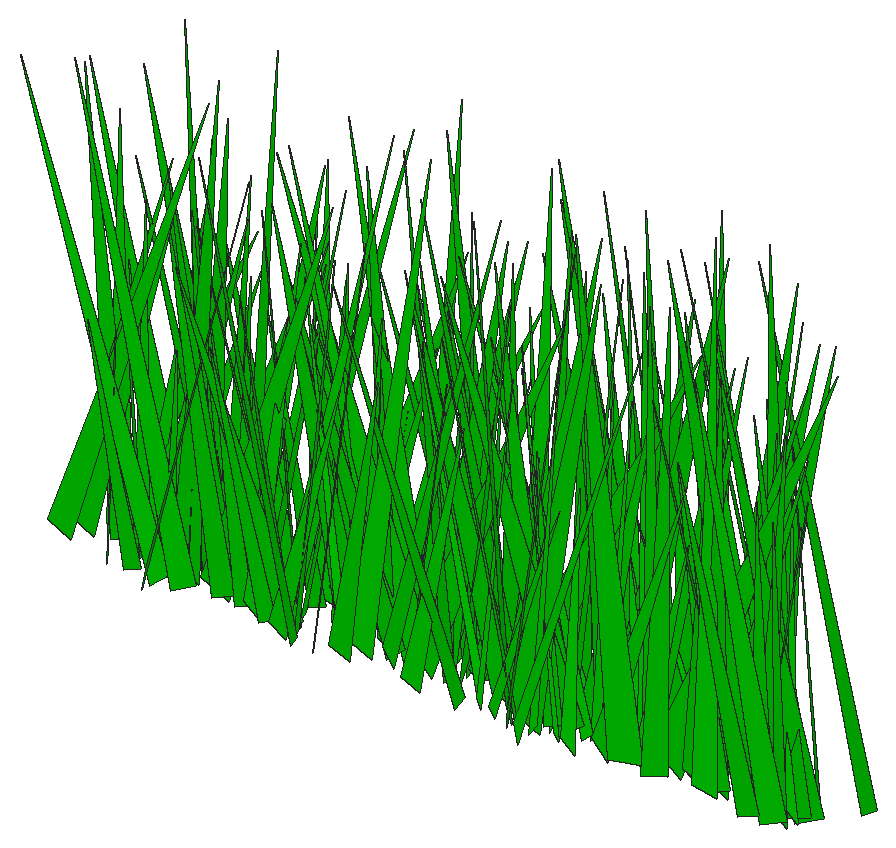
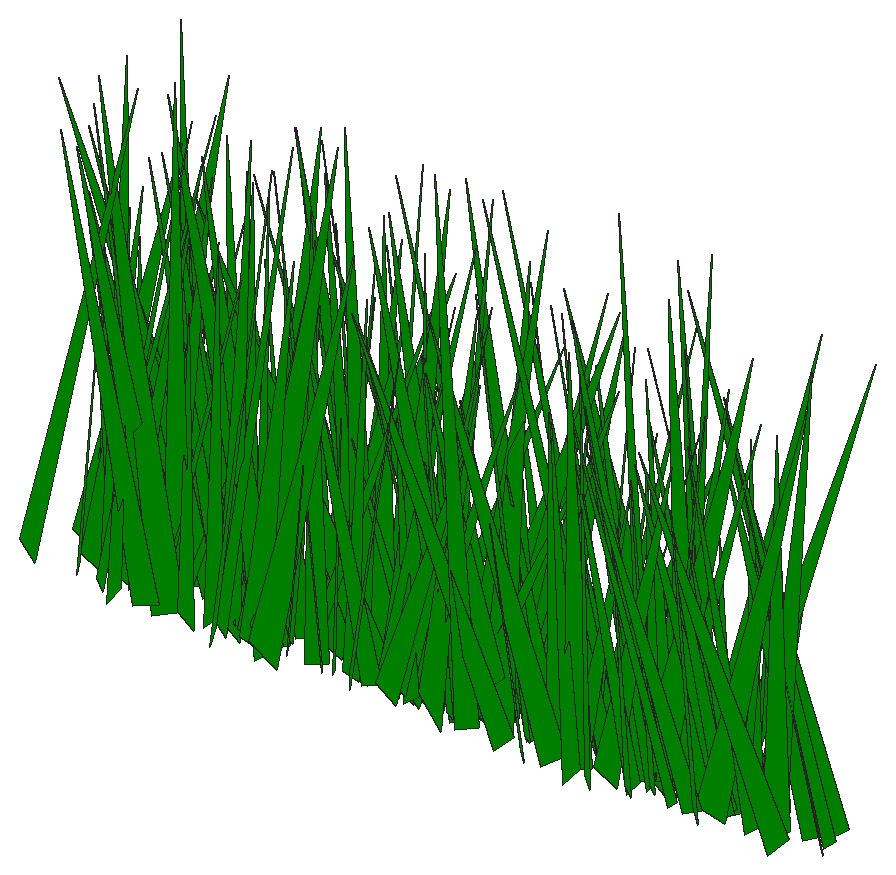
# SketchUp Ruby script. Lengths in inches.
U = 1.inch
M = Sketchup.active_model
def pt(a) = Geom::Point3d.new(a.map { |v| v * U })
def face(e, loops, mat)
  f = e.add_face(loops[0].map { |a| pt(a) })
  loops[1..].each { |l| e.add_face(l.map { |a| pt(a) }).erase! }
  f.material = f.back_material = mat if mat
  f
end
# faces: each face lists its corners as indices into pts; further lists are holes
def faces(e, pts, list, mat = nil) = list.each { |f| face(e, (f[0].is_a?(Array) ? f : [f]).map { |l| l.map { |i| pts[i] } }, mat) }
# xy, xz, yz: faces in a plane at the given z, y or x. An outline is a flat list of corners, or four numbers for a rectangle; further outlines are holes
def ring(l) = l.size == 4 ? [[l[0], l[1]], [l[2], l[1]], [l[2], l[3]], [l[0], l[3]]] : l.each_slice(2).to_a
def flat(e, list, mat, &to3) = list.each { |f| face(e, (f[0].is_a?(Array) ? f : [f]).map { |l| ring(l).map { |u, v| to3.(u, v) } }, mat) }
def xy(e, z, list, mat = nil) = flat(e, list, mat) { |x, y| [x, y, z] }
def xz(e, y, list, mat = nil) = flat(e, list, mat) { |x, z| [x, y, z] }
def yz(e, x, list, mat = nil) = flat(e, list, mat) { |y, z| [x, y, z] }
def lines(e, pts, list) = list.each { |a, b| e.add_line(pt(pts[a]), pt(pts[b])) }
# prism: a flat outline (further loops are holes) pulled along v
def prism(e, loops, v, mat = nil)
  f = face(e, loops, mat); d = Geom::Vector3d.new(v.map { |x| x * U })
  f.pushpull(f.normal.samedirection?(d) ? d.length : -d.length)
end
def box(e, o, s, mat = nil) = prism(e, [[o, [o[0] + s[0], o[1], o[2]], [o[0] + s[0], o[1] + s[1], o[2]], [o[0], o[1] + s[1], o[2]]]], [0, 0, s[2]], mat)
def at(x, y, z, deg = 0) = Geom::Transformation.translation(pt([x, y, z])) * Geom::Transformation.rotation(ORIGIN, Z_AXIS, deg.degrees)
def axes(o, x, y, z) = Geom::Transformation.new([*x, 0, *y, 0, *z, 0, *pt(o).to_a, 1])
def part(name) = M.definitions.add(name)
# library, detail: a bought-in or finely detailed component or shape, given as its bounding box
def library(name, o, s) = part(name).tap { |d| box(d.entities, o, s) }
def detail(e, o, s) = box(e.add_group.entities, o, s)
def put(e, d, t, mat = nil) = e.add_instance(d, t).tap { |i| i.material = mat if mat }
def group(e, t, mat = nil) = e.add_group.tap { |g| g.transformation = t; g.material = mat if mat }.entities
root = M.entities
M.materials.add("[Color G06]").color = [0, 204, 0]
c1 = part("fur_instance\#9")
p = [[0.8125,0,1.79],[0.67,-0.02,1.48],[0,-0.11,0],[0,0.11,0]]
faces(c1.entities,p,[[0,1,2,3]])
put(root,c1,axes([55.65,20.28,4.28],[5.61176,-0.00622,0.34921],[-0.14128,-0.70615,3.62553],[-0.19138,0.33878,7.56339]),"[Color G06]")
put(root,c1,axes([63.89,20.69,4.28],[-1.33664,-0.51587,0.86368],[-3.66618,0.16293,-1.49476],[-0.76079,0.1212,5.68569]),"[Color G06]")
put(root,c1,axes([55.9,20.74,4.28],[4.3108,-0.15482,1.6127],[-0.90664,-0.61328,-1.34984],[-1.25499,-0.08875,6.51469]),"[Color G06]")
put(root,c1,axes([47.3,20.49,4.28],[-5.15813,-0.18361,1.00453],[-1.44862,0.69564,-2.00901],[0.29502,0.20549,7.69861]),"[Color G06]")
put(root,c1,axes([48.74,20.8,4.28],[0.17225,-0.51156,0.1782],[-3.56401,-0.01933,1.32048],[0.87758,0.0219,5.32773]),"[Color G06]")
put(root,c1,axes([48,20.52,4.28],[4.73065,0.13241,1.54713],[0.71615,-0.66359,1.63292],[-1.20847,0.1251,7.02403]),"[Color G06]")
put(root,c1,axes([53.32,20.63,4.28],[-4.30887,-0.30441,0.17963],[-2.05694,0.55189,-2.77676],[-0.74095,0.23817,6.66388]),"[Color G06]")
put(root,c1,axes([47.08,20.88,4.28],[4.48614,-0.06707,1.55056],[-0.25746,-0.62989,-1.46616],[-1.11418,-0.12451,6.58198]),"[Color G06]")
put(root,c1,axes([46.53,20.69,4.28],[0.75026,0.41935,1.10788],[2.96194,-0.06605,-1.60866],[0.90551,-0.13141,4.34404]),"[Color G06]")
put(root,c1,axes([55.15,20.92,4.28],[-4.31973,-0.08526,0.66097],[-0.48604,0.5885,1.6253],[0.57725,-0.14255,6.3147]),"[Color G06]")
put(root,c1,axes([51.49,20.62,4.28],[0.45427,0.46095,0.33324],[3.22252,-0.05419,-1.20236],[0.76931,-0.0452,4.83973]),"[Color G06]")
put(root,c1,axes([41.02,20.92,4.28],[0.00529,-0.41185,0.31234],[-2.84927,-0.00863,-1.2001],[-0.80534,0.02784,4.24799]),"[Color G06]")
put(root,c1,axes([55.37,20.98,4.28],[0.88434,-0.78848,1.13337],[-5.53577,-0.09273,2.23801],[1.37928,0.13338,8.25565]),"[Color G06]")
put(root,c1,axes([54.36,20.8,4.28],[3.21465,0.20526,0.11236],[1.45259,-0.43695,-1.1358],[0.2497,-0.10064,5.16075]),"[Color G06]")
put(root,c1,axes([54.79,21.05,4.28],[-5.26365,-0.27233,2.16245],[-1.53968,0.746,2.42055],[1.88061,-0.15146,8.03422]),"[Color G06]")
put(root,c1,axes([57.3,20.61,4.28],[-2.28428,0.34124,0.15276],[2.2093,0.29549,-2.03032],[1.05725,0.1198,4.57273]),"[Color G06]")
put(root,c1,axes([64.74,20.79,4.28],[-2.39866,0.57535,1.39354],[4.18961,0.30252,1.76062],[-0.58355,-0.19305,6.91228]),"[Color G06]")
put(root,c1,axes([55.04,20.64,4.28],[5.59181,0.12004,1.74329],[0.53958,-0.7739,2.25577],[-1.34554,0.18854,8.14939]),"[Color G06]")
put(root,c1,axes([42.04,20.89,4.28],[-5.16613,0.3965,0.44493],[2.81524,0.69058,2.32082],[-0.49811,-0.20925,8.50236]),"[Color G06]")
put(root,c1,axes([64.8,21.04,4.28],[-2.41934,-0.36314,0.96588],[-2.45088,0.34847,1.33747],[1.09206,-0.02243,5.14146]),"[Color G06]")
put(root,c1,axes([39.99,21.04,4.28],[2.759,-0.02582,1.41235],[0.23074,-0.37051,-1.78491],[-0.9349,-0.16764,3.72749]),"[Color G06]")
put(root,c1,axes([45.95,20.96,4.28],[-0.80124,-0.38674,1.36753],[-2.80921,0.06589,-1.53606],[-0.79847,0.15628,4.03194]),"[Color G06]")
put(root,c1,axes([58.15,21.03,4.28],[2.1391,0.40842,1.58272],[2.98875,-0.21882,-2.53657],[0.87582,-0.2508,4.79046]),"[Color G06]")
put(root,c1,axes([56.7,20.85,4.28],[-3.97973,0.08571,1.28356],[0.41777,0.55659,-1.37601],[0.96995,0.11194,5.85911]),"[Color G06]")
put(root,c1,axes([46.68,21.17,4.28],[-0.89508,-0.58485,0.36657],[-3.78361,0.09701,-2.85625],[-1.82622,0.08565,5.73798]),"[Color G06]")
put(root,c1,axes([46.57,21.24,4.28],[-3.50626,-0.26054,0.35264],[-1.72714,0.47259,1.75065],[0.75079,-0.12962,5.67404]),"[Color G06]")
put(root,c1,axes([42.85,20.96,4.28],[-4.44763,0.52183,0.98901],[3.79199,0.60006,1.72142],[-0.25002,-0.18192,8.51495]),"[Color G06]")
put(root,c1,axes([42.09,21.22,4.28],[2.18178,-0.28491,0.17533],[-1.94386,-0.29598,-1.21839],[-0.64003,-0.07228,4.29805]),"[Color G06]")
put(root,c1,axes([51.22,20.88,4.28],[3.49246,0.08027,1.19757],[0.31189,-0.47975,1.66235],[-0.93603,0.13965,5.0222]),"[Color G06]")
put(root,c1,axes([59.18,20.9,4.28],[-1.64292,0.77619,1.38526],[5.62633,0.215,1.06648],[-0.43267,-0.15154,8.60824]),"[Color G06]")
put(root,c1,axes([56.2,21.31,4.28],[1.60443,-0.42544,0.27175],[-2.92586,-0.22208,-1.35239],[-0.88365,-0.03716,4.97131]),"[Color G06]")
put(root,c1,axes([62.03,21.46,4.28],[-2.12246,-0.69425,0.10684],[-4.77895,0.28708,2.22678],[1.39763,-0.07267,7.77633]),"[Color G06]")
put(root,c1,axes([63.86,21.36,4.28],[1.73266,-0.48961,0.05886],[-3.44238,-0.23806,-1.12561],[-0.69251,-0.04164,5.74254]),"[Color G06]")
put(root,c1,axes([62.02,21.02,4.28],[-4.62222,0.50172,3.33718],[3.60616,0.708,-1.07058],[2.21963,-0.10547,8.68877]),"[Color G06]")
put(root,c1,axes([60.33,20.82,4.28],[2.69761,0.69746,0.4034],[4.86547,-0.37502,1.80669],[-1.19034,0.04774,8.29895]),"[Color G06]")
put(root,c1,axes([53.73,20.98,4.28],[3.75595,0.01506,1.78859],[-0.30501,-0.51779,1.93155],[-1.16223,0.18455,5.27325]),"[Color G06]")
put(root,c1,axes([56.15,21.41,4.28],[3.86433,-0.22613,2.6542],[-0.93166,-0.57285,-2.57665],[-2.2171,-0.15342,5.70892]),"[Color G06]")
put(root,c1,axes([41.58,20.76,4.28],[5.71193,0.21022,0.12641],[1.25923,-0.68869,4.46601],[-0.83317,0.40033,7.61644]),"[Color G06]")
put(root,c1,axes([59.6,21.06,4.28],[-0.26074,0.40833,0.28772],[2.762,0.04325,-1.46028],[0.99139,-0.01311,4.14399]),"[Color G06]")
put(root,c1,axes([62.22,21.32,4.28],[-2.93792,0.018,1.41968],[0.37253,0.41489,1.11768],[0.88328,-0.1151,4.25068]),"[Color G06]")
put(root,c1,axes([56.82,21.33,4.28],[-1.28633,-0.67458,1.94852],[-4.58192,0.08246,-3.47719],[-2.02678,0.24171,6.62418]),"[Color G06]")
put(root,c1,axes([63.68,21.42,4.28],[-0.49349,-0.82073,2.15549],[-5.86672,0.01418,-2.38023],[-1.5176,0.21208,8.50053]),"[Color G06]")
put(root,c1,axes([62.82,21.55,4.28],[-4.48563,-0.2189,0.08506],[-1.48344,0.59822,2.10515],[0.5166,-0.1829,6.78364]),"[Color G06]")
put(root,c1,axes([63.82,21.42,4.28],[-1.86421,-0.51691,2.17679],[-3.72029,0.30606,1.23205],[1.42184,0.12309,6.07773]),"[Color G06]")
put(root,c1,axes([61.25,21.45,4.28],[-1.87846,-0.52409,1.87914],[-3.73148,0.29925,1.25534],[1.335,0.09901,6.15294]),"[Color G06]")
put(root,c1,axes([64.43,21.36,4.28],[-2.62616,0.22216,0.88302],[1.69745,0.34985,1.16559],[0.07667,-0.13601,4.44033]),"[Color G06]")
put(root,c1,axes([43.61,21.48,4.28],[2.96375,-0.64317,0.31202],[-4.45622,-0.38943,2.33643],[1.20795,0.1414,7.85376]),"[Color G06]")
put(root,c1,axes([57.4,21.39,4.28],[-2.74803,0.19675,0.89037],[1.52701,0.36512,1.259],[0.11802,-0.14293,4.44188]),"[Color G06]")
put(root,c1,axes([58.16,21.24,4.28],[3.74184,-0.08389,2.17953],[-0.9711,-0.53502,1.3585],[-1.24319,0.16542,5.49896]),"[Color G06]")
put(root,c1,axes([48.65,21.1,4.28],[-4.03721,0.23845,0.39076],[1.52911,0.5352,-2.22827],[0.80892,0.1784,6.16237]),"[Color G06]")
put(root,c1,axes([44.87,21.25,4.28],[0.19346,0.43582,0.98213],[3.07001,-0.05068,1.23278],[-0.88036,-0.08097,4.51481]),"[Color G06]")
put(root,c1,axes([45.25,21.14,4.28],[-3.15577,0.41206,2.24324],[2.44662,0.48458,-2.53697],[2.23576,0.05133,5.94256]),"[Color G06]")
put(root,c1,axes([63.46,21.58,4.28],[-1.81765,-0.33868,0.19529],[-2.15854,0.23509,1.95916],[1.12107,-0.09647,4.08884]),"[Color G06]")
put(root,c1,axes([50.02,21.46,4.28],[5.35433,0.32082,1.08165],[2.411,-0.71839,-2.1824],[-0.06283,-0.22709,8.43206]),"[Color G06]")
put(root,c1,axes([44.05,21.32,4.28],[-0.12293,0.55646,1.69761],[3.97972,-0.02899,1.73551],[-1.17326,-0.15665,5.70905]),"[Color G06]")
put(root,c1,axes([48.63,21.61,4.28],[-0.16155,-0.70019,0.99485],[-4.85783,-0.00488,-2.15685],[-1.43448,0.09539,7.19209]),"[Color G06]")
put(root,c1,axes([57.63,21.59,4.28],[3.73523,-0.28247,1.29746],[-1.83874,-0.53076,-1.44965],[-1.21492,-0.06516,6.183]),"[Color G06]")
put(root,c1,axes([62.35,21.26,4.28],[0.02111,0.51721,0.59549],[3.5928,-0.01777,1.48862],[-1.00391,-0.05272,5.33997]),"[Color G06]")
put(root,c1,axes([37.9,21.45,4.28],[5.11414,-0.47354,0.18988],[-3.30816,-0.68643,2.37561],[0.77722,0.19415,8.86217]),"[Color G06]")
put(root,c1,axes([49.04,21.33,4.28],[4.66231,-0.43817,2.92819],[-3.62976,-0.62771,2.11946],[-0.73284,0.32141,8.13132]),"[Color G06]")
put(root,c1,axes([46.55,21.7,4.28],[-4.54195,-0.19641,1.67502],[-0.9896,0.6268,2.4491],[1.50354,-0.18078,6.6719]),"[Color G06]")
put(root,c1,axes([65.46,21.55,4.28],[-0.92927,-0.68011,2.24794],[-4.88799,0.05724,-2.52412],[-1.46874,0.2398,6.97803]),"[Color G06]")
put(root,c1,axes([44,21.58,4.28],[-2.28473,-0.54873,1.60005],[-4.07544,0.30098,-1.14162],[-0.1487,0.18221,6.70425]),"[Color G06]")
put(root,c1,axes([54.68,21.41,4.28],[2.23751,0.74061,1.71928],[5.3909,-0.28064,-1.7843],[0.68498,-0.21053,8.42665]),"[Color G06]")
put(root,c1,axes([59.48,21.5,4.28],[3.90321,0.43345,0.84755],[3.15967,-0.53524,-1.05889],[0.00509,-0.12654,7.3819]),"[Color G06]")
put(root,c1,axes([63.47,21.7,4.28],[3.79104,-0.03397,0.83479],[-0.1095,-0.52077,-1.3236],[-0.59944,-0.11971,5.52123]),"[Color G06]")
put(root,c1,axes([42.26,21.76,4.28],[-2.44193,-0.71308,2.61601],[-5.03726,0.39735,1.93898],[1.95951,0.13281,8.24456]),"[Color G06]")
put(root,c1,axes([65.12,21.5,4.28],[1.13555,0.5577,2.26576],[3.99544,-0.21638,1.64532],[-1.5265,-0.15147,5.99194]),"[Color G06]")
put(root,c1,axes([59.94,21.24,4.28],[3.28986,0.62468,0.83275],[4.10678,-0.45407,2.88774],[-1.87436,0.10156,7.78878]),"[Color G06]")
put(root,c1,axes([46.13,21.47,4.28],[5.98583,-0.19657,1.38164],[-1.59407,-0.81472,2.11115],[-0.54833,0.22264,8.94525]),"[Color G06]")
put(root,c1,axes([52.32,22.05,4.28],[5.52235,-0.22922,0.50519],[-1.21575,-0.65819,-4.6201],[-1.15682,-0.40251,7.26715]),"[Color G06]")
put(root,c1,axes([60.09,21.66,4.28],[3.61952,-0.67875,0.47765],[-4.47691,-0.44019,3.92252],[1.93704,0.25093,8.17323]),"[Color G06]")
put(root,c1,axes([53.17,21.73,4.28],[-4.58714,0.06709,1.15615],[0.64852,0.6294,1.55214],[0.63975,-0.157,6.7164]),"[Color G06]")
put(root,c1,axes([55.67,21.53,4.28],[0.5135,0.658,2.30373],[4.78725,-0.1228,1.64577],[-1.31318,-0.19038,6.90056]),"[Color G06]")
put(root,c1,axes([52.23,21.51,4.28],[-5.17584,-0.26756,2.85431],[-2.37222,0.72511,-1.80051],[1.30442,0.25701,8.05126]),"[Color G06]")
put(root,c1,axes([57.875,21.57,4.28],[2.86402,0.409,2.75848],[2.94962,-0.46297,1.04483],[-1.81909,-0.10676,6.03718]),"[Color G06]")
put(root,c1,axes([64.87,21.45,4.28],[-3.23194,0.28674,0.84721],[1.7224,0.43548,-2.25456],[1.2582,0.14041,5.26258]),"[Color G06]")
put(root,c1,axes([54.1,21.8,4.28],[-0.60878,-0.6236,1.72244],[-4.30459,0.01792,-2.65319],[-1.67251,0.18086,6.20164]),"[Color G06]")
put(root,c1,axes([40.78,21.64,4.28],[-2.64642,-0.09582,1.57106],[-0.97175,0.37283,-1.04419],[0.79554,0.13664,3.95078]),"[Color G06]")
put(root,c1,axes([61.74,21.78,4.28],[3.32498,-0.40014,0.34713],[-2.83967,-0.44771,1.47286],[0.4734,0.1248,6.39675]),"[Color G06]")
put(root,c1,axes([40.47,22,4.28],[3.6568,-0.35549,0.88385],[-2.25524,-0.49995,-2.25696],[-1.32761,-0.12988,6.26843]),"[Color G06]")
put(root,c1,axes([50.0625,21.74,4.28],[-3.1292,-0.47628,0.95727],[-3.31841,0.37386,-2.86246],[-1.03166,0.24209,6.30379]),"[Color G06]")
put(root,c1,axes([49.53,21.99,4.28],[-1.55879,-0.44,0.21758],[-3.06098,0.216,1.19409],[0.77972,-0.03166,5.12267]),"[Color G06]")
put(root,c1,axes([60.13,21.8,4.28],[2.15862,-0.24837,0.28909],[-1.7637,-0.28717,1.07549],[0.31489,0.09417,4.04204]),"[Color G06]")
put(root,c1,axes([60.67,21.73,4.28],[3.42331,0.564,0.56747],[3.94979,-0.44591,-2.31326],[0.94984,-0.17844,7.57416]),"[Color G06]")
put(root,c1,axes([46.06,21.98,4.28],[-4.4151,-0.08225,0.0559],[-0.56335,0.59756,1.61065],[0.17867,-0.14829,6.45955]),"[Color G06]")
put(root,c1,axes([57.07,21.9,4.28],[0.47656,-0.54723,1.88209],[-3.95591,-0.01114,1.86529],[1.15624,0.18742,5.6061]),"[Color G06]")
put(root,c1,axes([53.99,22.24,4.28],[-2.69831,-0.70226,0.06481],[-4.79133,0.36007,2.59766],[1.55157,-0.10939,8.13443]),"[Color G06]")
put(root,c1,axes([54.19,21.8,4.28],[2.53594,-0.13226,1.43709],[-1.20593,-0.35017,1.05137],[-0.60818,0.14286,3.90759]),"[Color G06]")
put(root,c1,axes([50.77,21.92,4.28],[1.96931,0.63466,2.53212],[4.35733,-0.11834,-4.16244],[2.14441,-0.34237,6.13252]),"[Color G06]")
put(root,c1,axes([42.39,21.78,4.28],[4.6706,0.06577,2.51531],[0.21981,-0.68639,1.1501],[-1.73393,0.09015,6.92115]),"[Color G06]")
put(root,c1,axes([56.15,22.04,4.28],[-0.55081,-0.59491,0.85815],[-4.13931,0.05103,-1.87044],[-1.18186,0.09852,6.15107]),"[Color G06]")
put(root,c1,axes([38.31,22,4.28],[2.23084,-0.50735,0.48648],[-3.53565,-0.28654,1.88856],[0.91785,0.12933,6.09252]),"[Color G06]")
put(root,c1,axes([56.53,21.74,4.28],[5.15306,0.03343,2.12732],[-0.12418,-0.72287,1.97673],[-1.43805,0.1822,7.45224]),"[Color G06]")
put(root,c1,axes([42.97,22.24,4.28],[2.25847,-0.5707,0.14972],[-3.90764,-0.30527,-2.00411],[-1.22066,-0.07865,6.69265]),"[Color G06]")
put(root,c1,axes([49.94,21.94,4.28],[-4.69627,0.40981,0.96238],[3.0071,0.63422,1.75452],[-0.09348,-0.18625,8.09192]),"[Color G06]")
put(root,c1,axes([50.8,21.9,4.28],[-3.23064,0.65661,0.88809],[4.49967,0.39188,3.28038],[-1.50927,-0.23716,7.87902]),"[Color G06]")
put(root,c1,axes([42.55,22.29,4.28],[-1.56115,-0.79247,0.42569],[-5.48622,0.22056,2.22422],[1.50971,-0.01798,8.52289]),"[Color G06]")
put(root,c1,axes([55.48,21.6,4.28],[4.10197,0.61119,0.57098],[4.12597,-0.55969,2.61],[-1.52737,0.12952,8.584]),"[Color G06]")
put(root,c1,axes([61.27,22.25,4.28],[3.8081,-0.25225,0.91252],[-1.42882,-0.50253,-2.639],[-1.26634,-0.19155,5.72173]),"[Color G06]")
put(root,c1,axes([43.78,21.99,4.28],[-3.89423,-0.37186,0.80133],[-2.71391,0.52239,-1.61267],[-0.18291,0.16607,6.86724]),"[Color G06]")
put(root,c1,axes([37.7,22.05,4.28],[4.30171,0.34217,0.81993],[2.49957,-0.56554,-2.18172],[0.27234,-0.21412,7.0728]),"[Color G06]")
put(root,c1,axes([43.09,21.92,4.28],[-5.07544,-0.36291,3.52525],[-3.06635,0.7397,-1.11391],[1.71287,0.24886,8.45163]),"[Color G06]")
put(root,c1,axes([46.6,21.82,4.28],[2.50554,0.1592,0.08138],[1.02403,-0.3208,1.6664],[-0.50771,0.13863,3.76265]),"[Color G06]")
put(root,c1,axes([48.44,22.21,4.28],[2.92296,-0.3714,0.5422],[-2.5825,-0.40874,-1.06507],[-0.74575,-0.04025,5.81343]),"[Color G06]")
put(root,c1,axes([54.3,22.02,4.28],[-4.56866,-0.40007,1.25026],[-2.98742,0.6171,-1.70083],[0.08005,0.19663,7.8815]),"[Color G06]")
put(root,c1,axes([44.28,21.76,4.28],[2.48931,0.43907,0.13475],[2.93262,-0.32889,2.0902],[-1.14977,0.11173,5.62304]),"[Color G06]")
put(root,c1,axes([61.36,22.16,4.28],[-2.95484,0.0674,0.08072],[0.47039,0.38427,1.60453],[-0.12358,-0.1489,4.17737]),"[Color G06]")
put(root,c1,axes([59.7,22.33,4.28],[-0.58183,-0.67073,0.41008],[-4.56905,0.08904,2.24957],[1.52798,0.01086,6.88294]),"[Color G06]")
put(root,c1,axes([39.73,22.19,4.28],[2.28587,-0.60516,3.01434],[-4.437,-0.38478,-1.35799],[-1.79287,0.18068,7.20398]),"[Color G06]")
put(root,c1,axes([54.92,21.875,4.28],[-4.05531,0.63138,2.23206],[4.29678,0.60247,-2.13899],[2.06616,-0.01366,8.82916]),"[Color G06]")
put(root,c1,axes([51.34,22.3,4.28],[-0.70019,-0.43701,0.37053],[-3.03187,0.10323,1.18916],[0.83119,0.00842,4.64974]),"[Color G06]")
put(root,c1,axes([51.15,22.4,4.28],[1.44164,-0.76738,0.06853],[-5.41163,-0.19647,1.56301],[1.00026,0.04304,8.35743]),"[Color G06]")
put(root,c1,axes([64.73,22.34,4.28],[0.92778,-0.43942,0.49137],[-2.96242,-0.13725,-1.60578],[-1.12356,-0.00097,4.6396]),"[Color G06]")
put(root,c1,axes([44.23,22.24,4.28],[5.11821,0.37553,3.44674],[3.13363,-0.74332,-1.0909],[-1.65868,-0.24552,8.57471]),"[Color G06]")
put(root,c1,axes([37.74,22.38,4.28],[4.47804,0.00019,0.21268],[0.04609,-0.59299,-2.10703],[-0.13464,-0.19669,6.35244]),"[Color G06]")
put(root,c1,axes([52.68,22.15,4.28],[1.12385,0.36291,0.43881],[2.47617,-0.13272,-1.55668],[0.85307,-0.09285,3.94044]),"[Color G06]")
put(root,c1,axes([59.8125,22.27,4.28],[3.89558,0.40451,1.65307],[3.09871,-0.52182,-1.64308],[-0.19068,-0.21583,7.07077]),"[Color G06]")
put(root,c1,axes([40.9,22.11,4.28],[-2.97624,0.22069,0.43964],[1.47192,0.40801,-1.26967],[0.65171,0.08635,4.87539]),"[Color G06]")
put(root,c1,axes([47.74,22.17,4.28],[0.32736,0.42292,0.46467],[2.96126,-0.03374,-1.1328],[0.72515,-0.05315,4.41618]),"[Color G06]")
put(root,c1,axes([43.56,22.03,4.28],[3.61531,0.4657,0.87508],[3.10917,-0.50296,2.05473],[-1.35241,0.08862,7.06312]),"[Color G06]")
put(root,c1,axes([57.75,22.16,4.28],[1.66717,0.49707,1.8249],[3.39207,-0.27906,1.80969],[-1.64058,-0.07185,5.5962]),"[Color G06]")
put(root,c1,axes([43.83,21.96,4.28],[-4.98879,0.15715,1.04855],[0.68534,0.63072,-3.57536],[1.13692,0.30938,6.7563]),"[Color G06]")
put(root,c1,axes([54.07,22.31,4.28],[2.71583,0.68897,1.30855],[4.32414,-0.25093,-4.86994],[2.54551,-0.30881,6.87661]),"[Color G06]")
put(root,c1,axes([44.8125,22.4,4.28],[4.99126,0.14082,1.21495],[1.16163,-0.68599,-1.52645],[-0.57548,-0.16338,7.4563]),"[Color G06]")
put(root,c1,axes([45.68,22.23,4.28],[5.14176,0.4996,0.60195],[3.60014,-0.70624,-1.35687],[0.19313,-0.13585,9.26751]),"[Color G06]")
put(root,c1,axes([63.38,22.37,4.28],[-3.68849,0.3441,1.70787],[2.69775,0.49681,1.516],[0.34221,-0.20766,6.45705]),"[Color G06]")
put(root,c1,axes([50.49,22.41,4.28],[-3.82527,0.55422,3.07565],[4.46472,0.4989,2.07645],[0.31263,-0.34348,7.97871]),"[Color G06]")
put(root,c1,axes([49.53,22.625,4.28],[0.72768,-0.76476,0.93508],[-5.46045,-0.11261,-1.08797],[-0.8078,0.0723,8.19665]),"[Color G06]")
put(root,c1,axes([40.875,22.21,4.28],[-0.61184,0.43774,0.46434],[2.9235,0.09526,-1.71167],[1.18489,-0.00901,4.463]),"[Color G06]")
put(root,c1,axes([64.51,22.24,4.28],[-6.0592,-0.14343,0.71472],[-1.11814,0.81622,-2.35791],[0.19083,0.22833,8.87768]),"[Color G06]")
put(root,c1,axes([63.78,22.19,4.28],[-1.72191,0.40277,0.38955],[2.69685,0.23793,-1.63136],[1.06661,0.04865,4.75366]),"[Color G06]")
put(root,c1,axes([51.5,22.57,4.28],[4.01655,0.05927,0.38153],[0.48812,-0.52361,-2.1349],[-0.08684,-0.20198,5.64642]),"[Color G06]")
put(root,c1,axes([50.68,22.57,4.28],[-3.68329,0.19502,0.046],[1.25431,0.45506,2.71526],[-0.61939,-0.2382,5.22504]),"[Color G06]")
put(root,c1,axes([61.96,22.32,4.28],[1.64534,0.63728,2.35633],[4.47921,-0.28833,1.9714],[-1.81878,-0.13357,6.9867]),"[Color G06]")
put(root,c1,axes([48.15,22.52,4.28],[2.63526,-0.3749,0.40723],[-2.67076,-0.35325,1.24743],[0.41163,0.10814,5.48656]),"[Color G06]")
put(root,c1,axes([41.2,22.42,4.28],[1.58012,0.49546,0.91852],[3.42987,-0.17765,-2.17186],[1.11263,-0.15599,5.3907]),"[Color G06]")
put(root,c1,axes([46.52,22.54,4.28],[-1.25033,-0.41291,1.11015],[-3.022,0.15154,-1.12801],[-0.43276,0.13477,4.66962]),"[Color G06]")
put(root,c1,axes([44.01,22.28,4.28],[1.14237,0.78033,2.18983],[5.08149,-0.23489,3.69371],[-2.76409,-0.10931,7.69554]),"[Color G06]")
put(root,c1,axes([41.05,22.6,4.28],[3.47651,0.34711,1.53007],[2.68921,-0.43825,-2.22759],[0.11205,-0.25166,5.98967]),"[Color G06]")
put(root,c1,axes([48.37,22.64,4.28],[4.79456,-0.07783,1.38067],[-0.40387,-0.67332,-1.22749],[-1.00091,-0.10114,7.10902]),"[Color G06]")
put(root,c1,axes([44.01,22.3,4.28],[0.92205,0.73632,0.5811],[5.19038,-0.11483,-1.68117],[1.0456,-0.07927,7.83291]),"[Color G06]")
put(root,c1,axes([52.4,22.3,4.28],[4.44228,0.34135,2.48724],[1.94635,-0.65216,2.51646],[-2.23011,0.11077,7.15073]),"[Color G06]")
put(root,c1,axes([59.05,22.21,4.28],[-4.17199,0.53018,0.72155],[3.53529,0.57079,-2.51905],[1.47998,0.13107,8.05134]),"[Color G06]")
put(root,c1,axes([43.7,22.71,4.28],[3.35971,-0.09246,1.18606],[-0.42395,-0.46625,-1.49271],[-0.94321,-0.11976,4.89567]),"[Color G06]")
put(root,c1,axes([56.36,22.71,4.28],[-5.1199,0.12651,0.02202],[0.87751,0.68738,2.09676],[-0.23081,-0.19297,7.48307]),"[Color G06]")
put(root,c1,axes([63.57,22.36,4.28],[1.83713,0.38973,0.02814],[2.64251,-0.24323,1.61064],[-0.91033,0.08047,4.73214]),"[Color G06]")
put(root,c1,axes([62.64,22.76,4.28],[-2.21883,-0.45478,1.78531],[-3.14242,0.34705,1.43172],[1.47936,0.05509,5.71895]),"[Color G06]")
put(root,c1,axes([53.34,22.51,4.28],[1.67022,0.75668,3.06389],[5.44883,-0.30668,2.06579],[-1.98943,-0.20471,8.23024]),"[Color G06]")
put(root,c1,axes([51.55,23.15,4.28],[4.15461,-0.56231,0.27925],[-3.25343,-0.48855,-4.88814],[-2.38972,-0.31246,7.14035]),"[Color G06]")
put(root,c1,axes([63.67,22.45,4.28],[2.60112,0.75184,2.19503],[5.35793,-0.39971,1.54489],[-1.58717,-0.1172,8.81252]),"[Color G06]")
put(root,c1,axes([52.43,22.9,4.28],[-1.76229,-0.41926,0.34704],[-2.72098,0.23724,2.0608],[1.30005,-0.07179,4.78365]),"[Color G06]")
put(root,c1,axes([53.39,22.78,4.28],[1.04831,-0.5236,1.90976],[-3.62136,-0.20153,-1.90681],[-1.61784,0.11182,5.50566]),"[Color G06]")
put(root,c1,axes([50.5,22.8125,4.28],[1.09173,-0.73512,1.47709],[-5.11566,-0.10045,2.70309],[1.61185,0.17911,7.57855]),"[Color G06]")
put(root,c1,axes([43.86,22.59,4.28],[4.12802,-0.09342,1.22049],[-0.8574,-0.56464,1.51314],[-0.61685,0.15968,6.06443]),"[Color G06]")
put(root,c1,axes([55.89,22.93,4.28],[-2.59062,-0.61844,1.44093],[-4.28483,0.3843,1.73971],[1.49629,0.02977,7.47668]),"[Color G06]")
put(root,c1,axes([47.5,22.41,4.28],[2.71756,0.4953,0.23048],[3.2817,-0.35988,2.40756],[-1.36754,0.12064,6.23547]),"[Color G06]")
put(root,c1,axes([39.38,22.42,4.28],[-2.70509,0.60098,0.24839],[4.20636,0.37366,-1.52843],[0.95318,0.05662,7.44983]),"[Color G06]")
put(root,c1,axes([52.65,22.86,4.28],[-3.76881,0.26745,1.32407],[2.09848,0.50317,1.66676],[0.24482,-0.19565,6.09649]),"[Color G06]")
put(root,c1,axes([51,22.92,4.28],[3.81237,-0.11336,1.35982],[-0.636,-0.53985,-1.18671],[-1.04121,-0.08529,5.70382]),"[Color G06]")
put(root,c1,axes([49.3125,22.51,4.28],[-1.52407,0.59075,0.46927],[3.72739,0.20828,-3.07911],[2.03778,0.06085,5.9831]),"[Color G06]")
put(root,c1,axes([58.29,22.95,4.28],[-0.01804,-0.79486,2.21925],[-5.66987,-0.05378,-2.31566],[-1.59655,0.19997,8.19857]),"[Color G06]")
put(root,c1,axes([54.65,22.9,4.28],[3.2476,-0.32706,2.36807],[-2.25961,-0.50209,-1.044],[-1.70461,0.04246,5.89552]),"[Color G06]")
put(root,c1,axes([51.98,22.85,4.28],[-2.33391,-0.4234,1.4252],[-3.18185,0.30708,-1.15951],[-0.06478,0.17118,5.605]),"[Color G06]")
put(root,c1,axes([45.21,22.99,4.28],[0.63148,-0.54476,1.18074],[-3.68926,-0.1221,-2.06389],[-1.50827,0.07058,5.54268]),"[Color G06]")
put(root,c1,axes([57.47,22.97,4.28],[2.76523,-0.75411,1.18015],[-5.36599,-0.3512,2.3052],[1.03712,0.19356,8.78035]),"[Color G06]")
put(root,c1,axes([52.45,22.84,4.28],[-3.72316,-0.36419,0.42969],[-2.5724,0.49109,-1.97469],[-0.53504,0.17316,6.50391]),"[Color G06]")
put(root,c1,axes([39.98,22.79,4.28],[3.73808,-0.24669,1.52225],[-1.99283,-0.5052,1.52637],[-0.44219,0.19144,5.98945]),"[Color G06]")
put(root,c1,axes([61.67,23.05,4.28],[5.24999,0.14929,1.9407],[1.38172,-0.721,-1.97788],[-0.96081,-0.22111,7.75989]),"[Color G06]")
put(root,c1,axes([57.12,22.72,4.28],[-2.77292,0.05024,0.94619],[-0.0201,0.34206,-2.21792],[0.72814,0.20076,3.54207]),"[Color G06]")
put(root,c1,axes([53.22,23.11,4.28],[0.03975,-0.51386,0.27635],[-3.34896,-0.01585,-2.30895],[-1.54855,0.02108,5.00052]),"[Color G06]")
put(root,c1,axes([55.19,23.03,4.28],[2.58639,0.02993,2.03934],[0.61955,-0.38613,-1.10411],[-1.23454,-0.13107,3.71838]),"[Color G06]")
put(root,c1,axes([41.51,22.78,4.28],[-3.30991,0.62341,0.1201],[4.4233,0.45448,1.30333],[-0.65371,-0.08126,8.21083]),"[Color G06]")
put(root,c1,axes([53.87,22.92,4.28],[1.84906,0.48462,1.21119],[3.52761,-0.22899,-1.50451],[0.53934,-0.16376,5.688]),"[Color G06]")
put(root,c1,axes([57.33,23.35,4.28],[-2.20597,-0.77665,0.83909],[-4.89768,0.30853,4.04324],[2.71066,-0.07458,7.98828]),"[Color G06]")
put(root,c1,axes([58.16,22.78,4.28],[-4.67745,0.28623,2.0824],[1.77018,0.67559,-1.7857],[1.73813,0.08223,7.42253]),"[Color G06]")
put(root,c1,axes([66.52,22.96,4.28],[-5.27233,-0.40302,1.347],[-3.02628,0.70853,-2.10685],[0.08309,0.23303,8.73569]),"[Color G06]")
put(root,c1,axes([64.76,22.82,4.28],[-3.91803,0.0541,1.50205],[0.04176,0.53584,-1.97372],[1.07648,0.17612,5.54355]),"[Color G06]")
put(root,c1,axes([42.72,23.03,4.28],[4.05656,0.273,0.2844],[1.93926,-0.5449,-1.70063],[0.3292,-0.15419,6.51363]),"[Color G06]")
put(root,c1,axes([63.65,23.22,4.28],[-5.83847,-0.00296,1.45542],[0.2526,0.79238,2.44836],[0.94071,-0.23112,8.37555]),"[Color G06]")
put(root,c1,axes([55.56,23.13,4.28],[3.38735,0.02312,1.38628],[0.39085,-0.47363,-1.2259],[-0.85736,-0.12457,4.91822]),"[Color G06]")
put(root,c1,axes([44.2,23.21,4.28],[2.70793,-0.13293,0.66858],[-0.73384,-0.36166,-1.62118],[-0.75521,-0.12522,3.97261]),"[Color G06]")
put(root,c1,axes([38.77,23.06,4.28],[2.94408,-0.49723,0.49997],[-3.22979,-0.34252,3.35169],[1.54756,0.23108,6.0439]),"[Color G06]")
put(root,c1,axes([58.1,23.01,4.28],[-2.61644,0.75161,2.21419],[5.56004,0.32637,1.94928],[-0.57721,-0.2632,8.74001]),"[Color G06]")
put(root,c1,axes([42,23,4.28],[2.47988,0.48095,0.05622],[3.30074,-0.32902,-1.88155],[1.00121,-0.10655,6.06377]),"[Color G06]")
put(root,c1,axes([60.38,23.37,4.28],[2.82299,-0.36337,0.33504],[-2.36243,-0.374,-2.13243],[-1.12235,-0.12676,5.33126]),"[Color G06]")
put(root,c1,axes([61.69,22.96,4.28],[-4.7966,-0.11824,0.73949],[-0.96146,0.63532,-2.26113],[0.19842,0.22023,6.91996]),"[Color G06]")
put(root,c1,axes([62.93,23.48,4.28],[-3.90448,-0.43299,0.74618],[-2.60227,0.50712,3.38784],[1.76604,-0.21003,6.64173]),"[Color G06]")
put(root,c1,axes([61.06,23.32,4.28],[-0.53413,-0.81419,1.92694],[-5.68855,0.1248,2.53544],[1.84217,0.14931,8.38806]),"[Color G06]")
put(root,c1,axes([44.1875,22.99,4.28],[3.48315,-0.20762,1.89277],[-1.90312,-0.44255,2.24651],[-0.44594,0.26693,5.19671]),"[Color G06]")
put(root,c1,axes([59.16,22.91,4.28],[3.57285,0.63321,2.35402],[4.2264,-0.54423,2.48826],[-2.28878,-0.0165,8.26943]),"[Color G06]")
put(root,c1,axes([59.28,23.13,4.28],[-5.39018,-0.29002,2.01464],[-2.29958,0.75305,-1.2901],[0.92441,0.18222,8.538]),"[Color G06]")
put(root,c1,axes([61.01,22.95,4.28],[3.19636,0.72506,1.94698],[5.11697,-0.47573,1.58679],[-1.59666,-0.07312,8.98302]),"[Color G06]")
put(root,c1,axes([59.76,22.85,4.28],[-3.84156,0.43729,0.38817],[2.83747,0.50611,-2.77],[1.36024,0.17924,6.8745]),"[Color G06]")
put(root,c1,axes([46.01,23.57,4.28],[-2.74818,-0.52432,0.23823],[-3.18743,0.33891,3.55222],[2.00086,-0.18025,5.98601]),"[Color G06]")
put(root,c1,axes([46.97,23.15,4.28],[1.38836,0.65297,1.78693],[4.44667,-0.10465,-3.32456],[1.89306,-0.23308,6.49865]),"[Color G06]")
put(root,c1,axes([59.2,23.58,4.28],[-5.58339,-0.2806,1.41401],[-1.49077,0.73694,3.6508],[1.64984,-0.28373,8.08407]),"[Color G06]")
put(root,c1,axes([61.39,22.9375,4.28],[-0.74747,0.77399,0.38853],[5.21498,0.11034,-2.84056],[1.91825,0.00161,7.87381]),"[Color G06]")
put(root,c1,axes([45.46,23.51,4.28],[-4.17276,-0.08351,3.25321],[0.2267,0.61914,2.47537],[2.24616,-0.21763,5.79376]),"[Color G06]")
put(root,c1,axes([48.73,23.26,4.28],[3.01803,0.56419,0.24529],[3.67008,-0.36906,-3.35237],[1.71097,-0.20355,6.75826]),"[Color G06]")
put(root,c1,axes([50.13,23.22,4.28],[-4.49746,0.46182,3.93976],[3.32246,0.71746,-1.18908],[2.62264,-0.11696,8.26249]),"[Color G06]")
put(root,c1,axes([54.49,23.15,4.28],[-4.1938,-0.03026,1.29077],[-0.51292,0.55605,-2.22526],[0.72791,0.2175,5.86861]),"[Color G06]")
put(root,c1,axes([47.85,23.52,4.28],[2.83508,-0.04033,0.5286],[-0.09631,-0.35577,-1.96463],[-0.44663,-0.17931,3.77907]),"[Color G06]")
put(root,c1,axes([41.8,23.13,4.28],[3.3649,0.21757,1.10442],[1.21599,-0.45893,2.11004],[-1.22549,0.14203,5.12615]),"[Color G06]")
put(root,c1,axes([57.42,23.51,4.28],[1.1098,-0.67849,2.17857],[-4.56527,-0.22445,-2.83516],[-2.22656,0.12202,6.89898]),"[Color G06]")
put(root,c1,axes([57.97,23.24,4.28],[-0.66363,0.63193,1.54788],[4.60695,0.06993,1.13249],[-0.62067,-0.15662,6.75093]),"[Color G06]")
put(root,c1,axes([61.87,23.34,4.28],[2.50181,0.61725,1.84899],[4.55937,-0.30852,-1.94878],[0.57989,-0.23724,7.34512]),"[Color G06]")
put(root,c1,axes([46.125,23.12,4.28],[-2.60301,0.62431,0.61671],[4.3536,0.3666,-1.58528],[1.12288,0.02589,7.57603]),"[Color G06]")
